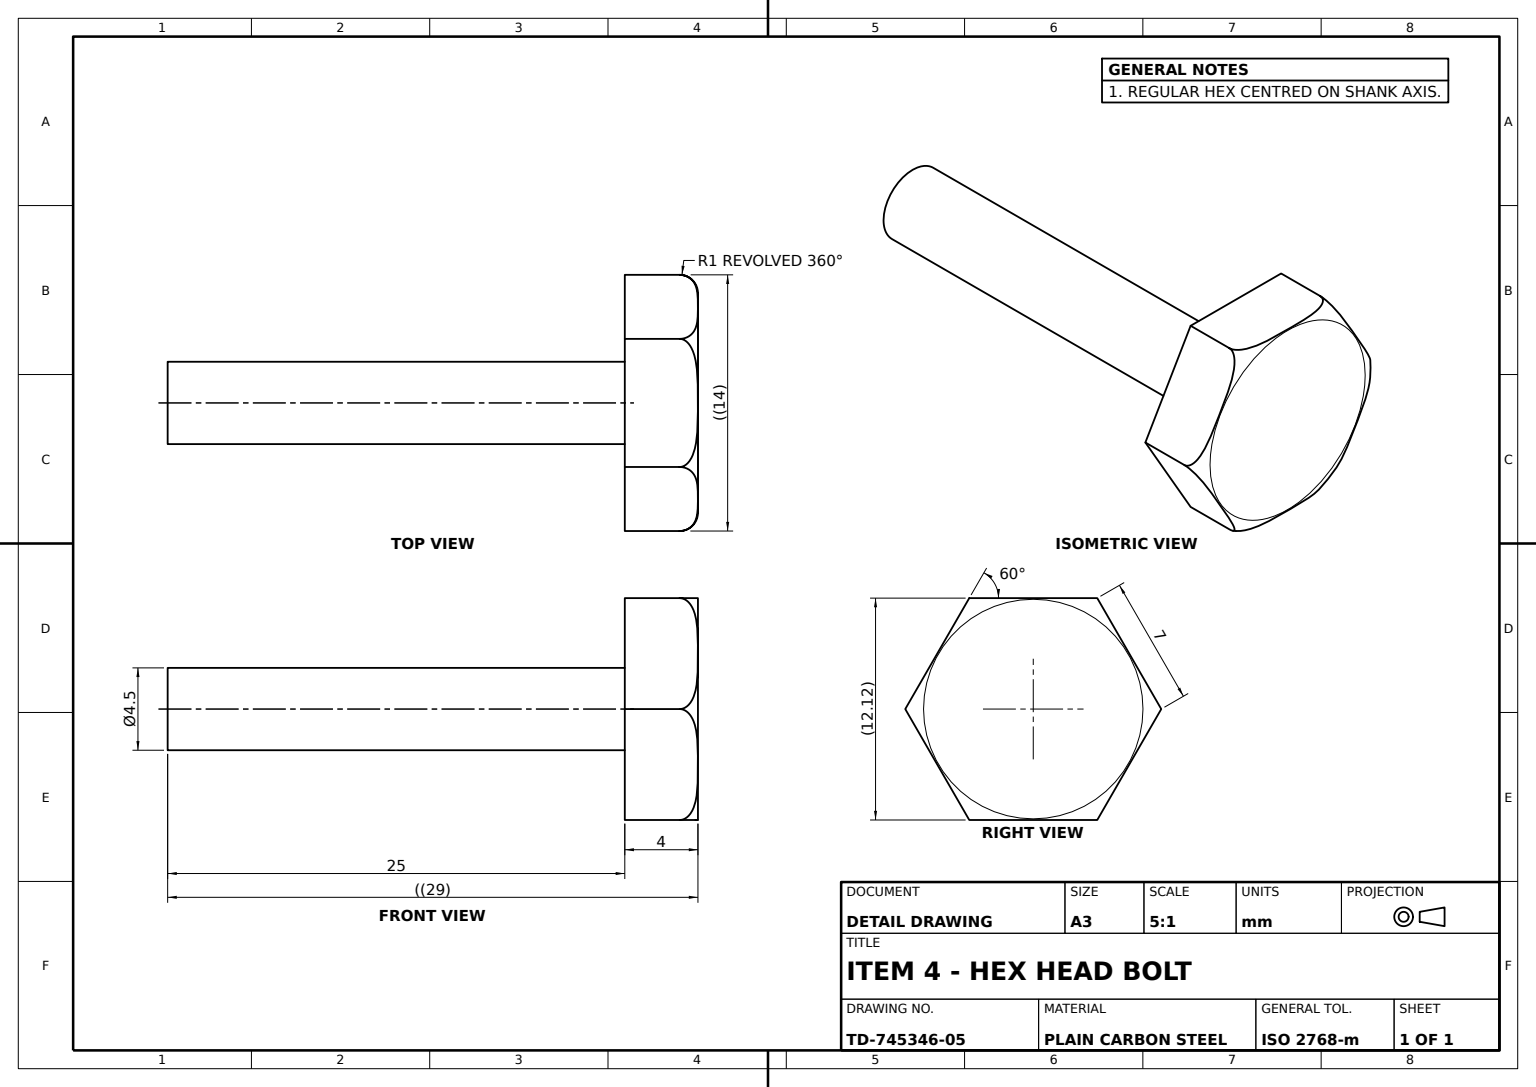
ISO-10303-21;
HEADER;
FILE_DESCRIPTION((''),'2;1');
FILE_NAME('','',(''),(''),'','','');
FILE_SCHEMA(('AUTOMOTIVE_DESIGN'));
ENDSEC;
DATA;
#1=APPLICATION_CONTEXT('');
#2=PRODUCT_CONTEXT('',#1,'mechanical');
#3=PRODUCT('','','',(#2));
#4=PRODUCT_DEFINITION_FORMATION('','',#3);
#5=PRODUCT_DEFINITION_CONTEXT('',#1,'design');
#6=PRODUCT_DEFINITION('','',#4,#5);
#7=PRODUCT_DEFINITION_SHAPE('','',#6);
#8=(LENGTH_UNIT()NAMED_UNIT(*)SI_UNIT(.MILLI.,.METRE.));
#9=(NAMED_UNIT(*)PLANE_ANGLE_UNIT()SI_UNIT($,.RADIAN.));
#10=(NAMED_UNIT(*)SI_UNIT($,.STERADIAN.)SOLID_ANGLE_UNIT());
#11=UNCERTAINTY_MEASURE_WITH_UNIT(LENGTH_MEASURE(1.E-05),#8,'distance_accuracy_value','');
#12=(GEOMETRIC_REPRESENTATION_CONTEXT(3)GLOBAL_UNCERTAINTY_ASSIGNED_CONTEXT((#11))GLOBAL_UNIT_ASSIGNED_CONTEXT((#8,#9,#10))REPRESENTATION_CONTEXT('',''));
#13=CARTESIAN_POINT('',(7.,0.,1.));
#14=VERTEX_POINT('',#13);
#15=CARTESIAN_POINT('',(3.5,-6.062178,1.));
#16=VERTEX_POINT('',#15);
#17=CARTESIAN_POINT('',(7.,0.,0.916819));
#18=CARTESIAN_POINT('',(6.989359,-0.018431,0.835633));
#19=CARTESIAN_POINT('',(6.952796,-0.081759,0.688304));
#20=CARTESIAN_POINT('',(6.92705,-0.126354,0.62203));
#21=CARTESIAN_POINT('',(6.868894,-0.227082,0.507162));
#22=CARTESIAN_POINT('',(6.835753,-0.284484,0.456904));
#23=CARTESIAN_POINT('',(6.766475,-0.404478,0.369773));
#24=CARTESIAN_POINT('',(6.730234,-0.467249,0.332584));
#25=CARTESIAN_POINT('',(6.618164,-0.661359,0.234345));
#26=CARTESIAN_POINT('',(6.539075,-0.798346,0.186761));
#27=CARTESIAN_POINT('',(6.381172,-1.071841,0.114066));
#28=CARTESIAN_POINT('',(6.3014,-1.210012,0.088523));
#29=CARTESIAN_POINT('',(6.060644,-1.627012,0.030791));
#30=CARTESIAN_POINT('',(5.89805,-1.908634,0.017016));
#31=CARTESIAN_POINT('',(5.573222,-2.471253,0.002538));
#32=CARTESIAN_POINT('',(5.41077,-2.752627,0.001924));
#33=CARTESIAN_POINT('',(5.08586,-3.315387,0.001946));
#34=CARTESIAN_POINT('',(4.923388,-3.596798,0.002584));
#35=CARTESIAN_POINT('',(4.598584,-4.159374,0.017273));
#36=CARTESIAN_POINT('',(4.436097,-4.44081,0.031131));
#37=CARTESIAN_POINT('',(4.194192,-4.859802,0.089809));
#38=CARTESIAN_POINT('',(4.113909,-4.998856,0.11589));
#39=CARTESIAN_POINT('',(3.956497,-5.271502,0.189267));
#40=CARTESIAN_POINT('',(3.879027,-5.405684,0.236251));
#41=CARTESIAN_POINT('',(3.729524,-5.66463,0.368438));
#42=CARTESIAN_POINT('',(3.65803,-5.788462,0.453009));
#43=CARTESIAN_POINT('',(3.571901,-5.937642,0.624608));
#44=CARTESIAN_POINT('',(3.546488,-5.981658,0.690617));
#45=CARTESIAN_POINT('',(3.510498,-6.043995,0.836797));
#46=CARTESIAN_POINT('',(3.5,-6.062178,0.917467));
#47=B_SPLINE_CURVE_WITH_KNOTS('',3,(#13,#17,#18,#19,#20,#21,#22,#23,#24,#25,#26,#27,#28,#29,#30,#31,#32,#33,#34,#35,#36,#37,#38,#39,#40,#41,#42,#43,#44,#45,#46,#15),.UNSPECIFIED.,.F.,.F.,(4,2,2,2,2,2,2,2,2,2,2,2,2,2,2,4),(0.000000197,0.000245943,0.000491689,0.000737435,0.000983181,0.001474674,0.001966166,0.00294915,0.003932135,0.004915119,0.005898103,0.006389596,0.006881088,0.00737258,0.007618326,0.007864072),.UNSPECIFIED.);
#48=EDGE_CURVE('',#14,#16,#47,.T.);
#49=ORIENTED_EDGE('',*,*,#48,.F.);
#50=CARTESIAN_POINT('',(7.,0.,4.));
#51=VERTEX_POINT('',#50);
#52=DIRECTION('',(0.,0.,-1.));
#53=VECTOR('',#52,1000.);
#54=LINE('',#50,#53);
#55=EDGE_CURVE('',#51,#14,#54,.T.);
#56=ORIENTED_EDGE('',*,*,#55,.F.);
#57=CARTESIAN_POINT('',(3.5,-6.062178,4.));
#58=VERTEX_POINT('',#57);
#59=DIRECTION('',(0.5,0.866025404,0.));
#60=VECTOR('',#59,1000.);
#61=LINE('',#57,#60);
#62=EDGE_CURVE('',#58,#51,#61,.T.);
#63=ORIENTED_EDGE('',*,*,#62,.F.);
#64=LINE('',#57,#53);
#65=EDGE_CURVE('',#58,#16,#64,.T.);
#66=ORIENTED_EDGE('',*,*,#65,.T.);
#67=EDGE_LOOP('',(#49,#56,#63,#66));
#68=FACE_OUTER_BOUND('',#67,.T.);
#69=DIRECTION('',(-0.866025404,0.5,0.));
#70=DIRECTION('',(-0.5,-0.866025404,0.));
#71=AXIS2_PLACEMENT_3D('',#57,#69,#70);
#72=PLANE('',#71);
#73=ADVANCED_FACE('',(#68),#72,.F.);
#74=CARTESIAN_POINT('',(-6.,0.,0.));
#75=VERTEX_POINT('',#74);
#76=CARTESIAN_POINT('',(6.,0.,0.));
#77=VERTEX_POINT('',#76);
#78=CARTESIAN_POINT('',(0.,0.,0.));
#79=DIRECTION('',(-1.,0.,0.));
#80=AXIS2_PLACEMENT_3D('',#78,#52,#79);
#81=CIRCLE('',#80,6.);
#82=EDGE_CURVE('',#75,#77,#81,.T.);
#83=ORIENTED_EDGE('',*,*,#82,.F.);
#84=CARTESIAN_POINT('',(-7.,0.,1.));
#85=VERTEX_POINT('',#84);
#86=CARTESIAN_POINT('',(-6.,0.,1.));
#87=DIRECTION('',(0.,-1.,0.));
#88=AXIS2_PLACEMENT_3D('',#86,#87,#52);
#89=CIRCLE('',#88,1.);
#90=EDGE_CURVE('',#85,#75,#89,.T.);
#91=ORIENTED_EDGE('',*,*,#90,.F.);
#92=CARTESIAN_POINT('',(-3.5,6.062178,1.));
#93=VERTEX_POINT('',#92);
#94=CARTESIAN_POINT('',(-7.,0.,0.916819));
#95=CARTESIAN_POINT('',(-6.989359,0.018431,0.835633));
#96=CARTESIAN_POINT('',(-6.952796,0.081759,0.688304));
#97=CARTESIAN_POINT('',(-6.92705,0.126354,0.62203));
#98=CARTESIAN_POINT('',(-6.868894,0.227082,0.507162));
#99=CARTESIAN_POINT('',(-6.835753,0.284484,0.456904));
#100=CARTESIAN_POINT('',(-6.766475,0.404478,0.369773));
#101=CARTESIAN_POINT('',(-6.730234,0.467249,0.332584));
#102=CARTESIAN_POINT('',(-6.618164,0.661359,0.234345));
#103=CARTESIAN_POINT('',(-6.539075,0.798346,0.186761));
#104=CARTESIAN_POINT('',(-6.381172,1.071841,0.114066));
#105=CARTESIAN_POINT('',(-6.3014,1.210012,0.088523));
#106=CARTESIAN_POINT('',(-6.060644,1.627012,0.030791));
#107=CARTESIAN_POINT('',(-5.89805,1.908634,0.017016));
#108=CARTESIAN_POINT('',(-5.573222,2.471253,0.002538));
#109=CARTESIAN_POINT('',(-5.41077,2.752627,0.001924));
#110=CARTESIAN_POINT('',(-5.08586,3.315387,0.001946));
#111=CARTESIAN_POINT('',(-4.923388,3.596798,0.002584));
#112=CARTESIAN_POINT('',(-4.598584,4.159374,0.017273));
#113=CARTESIAN_POINT('',(-4.436097,4.44081,0.031131));
#114=CARTESIAN_POINT('',(-4.194192,4.859802,0.089809));
#115=CARTESIAN_POINT('',(-4.113909,4.998856,0.11589));
#116=CARTESIAN_POINT('',(-3.956497,5.271502,0.189267));
#117=CARTESIAN_POINT('',(-3.879027,5.405684,0.236251));
#118=CARTESIAN_POINT('',(-3.729524,5.66463,0.368438));
#119=CARTESIAN_POINT('',(-3.65803,5.788462,0.453009));
#120=CARTESIAN_POINT('',(-3.571901,5.937642,0.624608));
#121=CARTESIAN_POINT('',(-3.546488,5.981658,0.690617));
#122=CARTESIAN_POINT('',(-3.510498,6.043995,0.836797));
#123=CARTESIAN_POINT('',(-3.5,6.062178,0.917467));
#124=B_SPLINE_CURVE_WITH_KNOTS('',3,(#84,#94,#95,#96,#97,#98,#99,#100,#101,#102,#103,#104,#105,#106,#107,#108,#109,#110,#111,#112,#113,#114,#115,#116,#117,#118,#119,#120,#121,#122,#123,#92),.UNSPECIFIED.,.F.,.F.,(4,2,2,2,2,2,2,2,2,2,2,2,2,2,2,4),(0.000000197,0.000245943,0.000491689,0.000737435,0.000983181,0.001474674,0.001966166,0.00294915,0.003932135,0.004915119,0.005898103,0.006389596,0.006881088,0.00737258,0.007618326,0.007864072),.UNSPECIFIED.);
#125=EDGE_CURVE('',#85,#93,#124,.T.);
#126=ORIENTED_EDGE('',*,*,#125,.T.);
#127=CARTESIAN_POINT('',(3.5,6.062178,1.));
#128=VERTEX_POINT('',#127);
#129=CARTESIAN_POINT('',(-3.5,6.062178,0.918745));
#130=CARTESIAN_POINT('',(-3.479253,6.062178,0.837184));
#131=CARTESIAN_POINT('',(-3.406434,6.062178,0.689536));
#132=CARTESIAN_POINT('',(-3.356443,6.062178,0.624754));
#133=CARTESIAN_POINT('',(-3.181801,6.062178,0.451074));
#134=CARTESIAN_POINT('',(-3.039481,6.062178,0.367715));
#135=CARTESIAN_POINT('',(-2.741948,6.062178,0.236325));
#136=CARTESIAN_POINT('',(-2.587351,6.062178,0.189346));
#137=CARTESIAN_POINT('',(-2.271801,6.062178,0.115802));
#138=CARTESIAN_POINT('',(-2.110688,6.062178,0.08969));
#139=CARTESIAN_POINT('',(-1.628975,6.062178,0.031285));
#140=CARTESIAN_POINT('',(-1.306565,6.062178,0.01745));
#141=CARTESIAN_POINT('',(-0.661096,6.062178,0.002671));
#142=CARTESIAN_POINT('',(-0.338023,6.062178,0.001986));
#143=CARTESIAN_POINT('',(0.146635,6.062178,0.001911));
#144=CARTESIAN_POINT('',(0.310793,6.062178,0.002231));
#145=CARTESIAN_POINT('',(0.636565,6.062178,0.004285));
#146=CARTESIAN_POINT('',(0.799424,6.062178,0.00602));
#147=CARTESIAN_POINT('',(1.287798,6.062178,0.016692));
#148=CARTESIAN_POINT('',(1.613148,6.062178,0.03008));
#149=CARTESIAN_POINT('',(2.09976,6.062178,0.088029));
#150=CARTESIAN_POINT('',(2.260961,6.062178,0.11381));
#151=CARTESIAN_POINT('',(2.576967,6.062178,0.186427));
#152=CARTESIAN_POINT('',(2.73221,6.062178,0.232886));
#153=CARTESIAN_POINT('',(3.032378,6.062178,0.363764));
#154=CARTESIAN_POINT('',(3.176959,6.062178,0.447407));
#155=CARTESIAN_POINT('',(3.354082,6.062178,0.621855));
#156=CARTESIAN_POINT('',(3.405203,6.062178,0.68762));
#157=CARTESIAN_POINT('',(3.478814,6.062178,0.835728));
#158=CARTESIAN_POINT('',(3.5,6.062178,0.918017));
#159=B_SPLINE_CURVE_WITH_KNOTS('',3,(#92,#129,#130,#131,#132,#133,#134,#135,#136,#137,#138,#139,#140,#141,#142,#143,#144,#145,#146,#147,#148,#149,#150,#151,#152,#153,#154,#155,#156,#157,#158,#127),.UNSPECIFIED.,.F.,.F.,(4,2,2,2,2,2,2,2,2,2,2,2,2,2,2,4),(0.011690306,0.011934522,0.012178739,0.012667172,0.013155605,0.013644038,0.014620904,0.01559777,0.016086203,0.016574636,0.017551502,0.018039935,0.018528368,0.019016801,0.019261017,0.019505234),.UNSPECIFIED.);
#160=EDGE_CURVE('',#93,#128,#159,.T.);
#161=ORIENTED_EDGE('',*,*,#160,.T.);
#162=CARTESIAN_POINT('',(3.5,6.062178,0.916819));
#163=CARTESIAN_POINT('',(3.510641,6.043747,0.835633));
#164=CARTESIAN_POINT('',(3.547204,5.980418,0.688304));
#165=CARTESIAN_POINT('',(3.57295,5.935824,0.62203));
#166=CARTESIAN_POINT('',(3.631106,5.835096,0.507162));
#167=CARTESIAN_POINT('',(3.664247,5.777694,0.456904));
#168=CARTESIAN_POINT('',(3.733525,5.6577,0.369773));
#169=CARTESIAN_POINT('',(3.769766,5.594929,0.332584));
#170=CARTESIAN_POINT('',(3.881836,5.400819,0.234345));
#171=CARTESIAN_POINT('',(3.960925,5.263832,0.186761));
#172=CARTESIAN_POINT('',(4.118828,4.990337,0.114066));
#173=CARTESIAN_POINT('',(4.1986,4.852166,0.088523));
#174=CARTESIAN_POINT('',(4.439356,4.435166,0.030791));
#175=CARTESIAN_POINT('',(4.60195,4.153544,0.017016));
#176=CARTESIAN_POINT('',(4.926778,3.590925,0.002538));
#177=CARTESIAN_POINT('',(5.08923,3.309551,0.001924));
#178=CARTESIAN_POINT('',(5.41414,2.746791,0.001946));
#179=CARTESIAN_POINT('',(5.576612,2.46538,0.002584));
#180=CARTESIAN_POINT('',(5.901416,1.902804,0.017273));
#181=CARTESIAN_POINT('',(6.063903,1.621368,0.031131));
#182=CARTESIAN_POINT('',(6.305808,1.202376,0.089809));
#183=CARTESIAN_POINT('',(6.386091,1.063322,0.11589));
#184=CARTESIAN_POINT('',(6.543503,0.790676,0.189267));
#185=CARTESIAN_POINT('',(6.620973,0.656494,0.236251));
#186=CARTESIAN_POINT('',(6.770476,0.397548,0.368438));
#187=CARTESIAN_POINT('',(6.84197,0.273716,0.453009));
#188=CARTESIAN_POINT('',(6.928099,0.124536,0.624608));
#189=CARTESIAN_POINT('',(6.953512,0.080519,0.690617));
#190=CARTESIAN_POINT('',(6.989502,0.018183,0.836797));
#191=CARTESIAN_POINT('',(7.,0.,0.917467));
#192=B_SPLINE_CURVE_WITH_KNOTS('',3,(#127,#162,#163,#164,#165,#166,#167,#168,#169,#170,#171,#172,#173,#174,#175,#176,#177,#178,#179,#180,#181,#182,#183,#184,#185,#186,#187,#188,#189,#190,#191,#13),.UNSPECIFIED.,.F.,.F.,(4,2,2,2,2,2,2,2,2,2,2,2,2,2,2,4),(0.000000197,0.000245943,0.000491689,0.000737435,0.000983181,0.001474674,0.001966166,0.00294915,0.003932135,0.004915119,0.005898103,0.006389596,0.006881088,0.00737258,0.007618326,0.007864072),.UNSPECIFIED.);
#193=EDGE_CURVE('',#128,#14,#192,.T.);
#194=ORIENTED_EDGE('',*,*,#193,.T.);
#195=CARTESIAN_POINT('',(6.,0.,1.));
#196=DIRECTION('',(0.,1.,0.));
#197=AXIS2_PLACEMENT_3D('',#195,#196,#79);
#198=CIRCLE('',#197,1.);
#199=EDGE_CURVE('',#14,#77,#198,.T.);
#200=ORIENTED_EDGE('',*,*,#199,.T.);
#201=EDGE_LOOP('',(#83,#91,#126,#161,#194,#200));
#202=FACE_OUTER_BOUND('',#201,.T.);
#203=CARTESIAN_POINT('',(0.,0.,1.));
#204=AXIS2_PLACEMENT_3D('',#203,#52,#79);
#205=TOROIDAL_SURFACE('',#204,6.,1.);
#206=ADVANCED_FACE('',(#202),#205,.T.);
#207=CARTESIAN_POINT('',(3.5,6.062178,4.));
#208=VERTEX_POINT('',#207);
#209=LINE('',#207,#53);
#210=EDGE_CURVE('',#208,#128,#209,.T.);
#211=ORIENTED_EDGE('',*,*,#210,.T.);
#212=ORIENTED_EDGE('',*,*,#160,.F.);
#213=CARTESIAN_POINT('',(-3.5,6.062178,4.));
#214=VERTEX_POINT('',#213);
#215=LINE('',#213,#53);
#216=EDGE_CURVE('',#214,#93,#215,.T.);
#217=ORIENTED_EDGE('',*,*,#216,.F.);
#218=VECTOR('',#79,1000.);
#219=LINE('',#207,#218);
#220=EDGE_CURVE('',#208,#214,#219,.T.);
#221=ORIENTED_EDGE('',*,*,#220,.F.);
#222=EDGE_LOOP('',(#211,#212,#217,#221));
#223=FACE_OUTER_BOUND('',#222,.T.);
#224=AXIS2_PLACEMENT_3D('',#207,#87,#52);
#225=PLANE('',#224);
#226=ADVANCED_FACE('',(#223),#225,.F.);
#227=ORIENTED_EDGE('',*,*,#193,.F.);
#228=ORIENTED_EDGE('',*,*,#210,.F.);
#229=DIRECTION('',(-0.5,0.866025404,0.));
#230=VECTOR('',#229,1000.);
#231=LINE('',#50,#230);
#232=EDGE_CURVE('',#51,#208,#231,.T.);
#233=ORIENTED_EDGE('',*,*,#232,.F.);
#234=ORIENTED_EDGE('',*,*,#55,.T.);
#235=EDGE_LOOP('',(#227,#228,#233,#234));
#236=FACE_OUTER_BOUND('',#235,.T.);
#237=DIRECTION('',(-0.866025404,-0.5,0.));
#238=DIRECTION('',(0.5,-0.866025404,0.));
#239=AXIS2_PLACEMENT_3D('',#50,#237,#238);
#240=PLANE('',#239);
#241=ADVANCED_FACE('',(#236),#240,.F.);
#242=CARTESIAN_POINT('',(-2.25,0.,29.));
#243=VERTEX_POINT('',#242);
#244=CARTESIAN_POINT('',(2.25,0.,29.));
#245=VERTEX_POINT('',#244);
#246=CARTESIAN_POINT('',(0.,0.,29.));
#247=DIRECTION('',(0.,0.,1.));
#248=DIRECTION('',(1.,0.,0.));
#249=AXIS2_PLACEMENT_3D('',#246,#247,#248);
#250=CIRCLE('',#249,2.25);
#251=EDGE_CURVE('',#243,#245,#250,.T.);
#252=ORIENTED_EDGE('',*,*,#251,.T.);
#253=EDGE_CURVE('',#245,#243,#250,.T.);
#254=ORIENTED_EDGE('',*,*,#253,.T.);
#255=EDGE_LOOP('',(#252,#254));
#256=FACE_OUTER_BOUND('',#255,.T.);
#257=PLANE('',#249);
#258=ADVANCED_FACE('',(#256),#257,.T.);
#259=ORIENTED_EDGE('',*,*,#65,.F.);
#260=CARTESIAN_POINT('',(-3.5,-6.062178,4.));
#261=VERTEX_POINT('',#260);
#262=VECTOR('',#248,1000.);
#263=LINE('',#260,#262);
#264=EDGE_CURVE('',#261,#58,#263,.T.);
#265=ORIENTED_EDGE('',*,*,#264,.F.);
#266=CARTESIAN_POINT('',(-3.5,-6.062178,1.));
#267=VERTEX_POINT('',#266);
#268=LINE('',#260,#53);
#269=EDGE_CURVE('',#261,#267,#268,.T.);
#270=ORIENTED_EDGE('',*,*,#269,.T.);
#271=CARTESIAN_POINT('',(3.5,-6.062178,0.918745));
#272=CARTESIAN_POINT('',(3.479253,-6.062178,0.837184));
#273=CARTESIAN_POINT('',(3.406434,-6.062178,0.689536));
#274=CARTESIAN_POINT('',(3.356443,-6.062178,0.624754));
#275=CARTESIAN_POINT('',(3.181801,-6.062178,0.451074));
#276=CARTESIAN_POINT('',(3.039481,-6.062178,0.367715));
#277=CARTESIAN_POINT('',(2.741948,-6.062178,0.236325));
#278=CARTESIAN_POINT('',(2.587351,-6.062178,0.189346));
#279=CARTESIAN_POINT('',(2.271801,-6.062178,0.115802));
#280=CARTESIAN_POINT('',(2.110688,-6.062178,0.08969));
#281=CARTESIAN_POINT('',(1.628975,-6.062178,0.031285));
#282=CARTESIAN_POINT('',(1.306565,-6.062178,0.01745));
#283=CARTESIAN_POINT('',(0.661096,-6.062178,0.002671));
#284=CARTESIAN_POINT('',(0.338023,-6.062178,0.001986));
#285=CARTESIAN_POINT('',(-0.146635,-6.062178,0.001911));
#286=CARTESIAN_POINT('',(-0.310793,-6.062178,0.002231));
#287=CARTESIAN_POINT('',(-0.636565,-6.062178,0.004285));
#288=CARTESIAN_POINT('',(-0.799424,-6.062178,0.00602));
#289=CARTESIAN_POINT('',(-1.287798,-6.062178,0.016692));
#290=CARTESIAN_POINT('',(-1.613148,-6.062178,0.03008));
#291=CARTESIAN_POINT('',(-2.09976,-6.062178,0.088029));
#292=CARTESIAN_POINT('',(-2.260961,-6.062178,0.11381));
#293=CARTESIAN_POINT('',(-2.576967,-6.062178,0.186427));
#294=CARTESIAN_POINT('',(-2.73221,-6.062178,0.232886));
#295=CARTESIAN_POINT('',(-3.032378,-6.062178,0.363764));
#296=CARTESIAN_POINT('',(-3.176959,-6.062178,0.447407));
#297=CARTESIAN_POINT('',(-3.354082,-6.062178,0.621855));
#298=CARTESIAN_POINT('',(-3.405203,-6.062178,0.68762));
#299=CARTESIAN_POINT('',(-3.478814,-6.062178,0.835728));
#300=CARTESIAN_POINT('',(-3.5,-6.062178,0.918017));
#301=B_SPLINE_CURVE_WITH_KNOTS('',3,(#15,#271,#272,#273,#274,#275,#276,#277,#278,#279,#280,#281,#282,#283,#284,#285,#286,#287,#288,#289,#290,#291,#292,#293,#294,#295,#296,#297,#298,#299,#300,#266),.UNSPECIFIED.,.F.,.F.,(4,2,2,2,2,2,2,2,2,2,2,2,2,2,2,4),(0.011690306,0.011934522,0.012178739,0.012667172,0.013155605,0.013644038,0.014620904,0.01559777,0.016086203,0.016574636,0.017551502,0.018039935,0.018528368,0.019016801,0.019261017,0.019505234),.UNSPECIFIED.);
#302=EDGE_CURVE('',#16,#267,#301,.T.);
#303=ORIENTED_EDGE('',*,*,#302,.F.);
#304=EDGE_LOOP('',(#259,#265,#270,#303));
#305=FACE_OUTER_BOUND('',#304,.T.);
#306=AXIS2_PLACEMENT_3D('',#260,#196,#79);
#307=PLANE('',#306);
#308=ADVANCED_FACE('',(#305),#307,.F.);
#309=CARTESIAN_POINT('',(-2.25,0.,4.));
#310=VERTEX_POINT('',#309);
#311=CARTESIAN_POINT('',(2.25,0.,4.));
#312=VERTEX_POINT('',#311);
#313=CARTESIAN_POINT('',(0.,0.,4.));
#314=AXIS2_PLACEMENT_3D('',#313,#247,#248);
#315=CIRCLE('',#314,2.25);
#316=EDGE_CURVE('',#310,#312,#315,.T.);
#317=ORIENTED_EDGE('',*,*,#316,.F.);
#318=EDGE_CURVE('',#312,#310,#315,.T.);
#319=ORIENTED_EDGE('',*,*,#318,.F.);
#320=EDGE_LOOP('',(#317,#319));
#321=FACE_BOUND('',#320,.T.);
#322=CARTESIAN_POINT('',(-7.,0.,4.));
#323=VERTEX_POINT('',#322);
#324=VECTOR('',#70,1000.);
#325=LINE('',#213,#324);
#326=EDGE_CURVE('',#214,#323,#325,.T.);
#327=ORIENTED_EDGE('',*,*,#326,.T.);
#328=VECTOR('',#238,1000.);
#329=LINE('',#322,#328);
#330=EDGE_CURVE('',#323,#261,#329,.T.);
#331=ORIENTED_EDGE('',*,*,#330,.T.);
#332=ORIENTED_EDGE('',*,*,#264,.T.);
#333=ORIENTED_EDGE('',*,*,#62,.T.);
#334=ORIENTED_EDGE('',*,*,#232,.T.);
#335=ORIENTED_EDGE('',*,*,#220,.T.);
#336=EDGE_LOOP('',(#327,#331,#332,#333,#334,#335));
#337=FACE_OUTER_BOUND('',#336,.T.);
#338=PLANE('',#314);
#339=ADVANCED_FACE('',(#321,#337),#338,.T.);
#340=ORIENTED_EDGE('',*,*,#302,.T.);
#341=CARTESIAN_POINT('',(-3.5,-6.062178,0.916819));
#342=CARTESIAN_POINT('',(-3.510641,-6.043747,0.835633));
#343=CARTESIAN_POINT('',(-3.547204,-5.980418,0.688304));
#344=CARTESIAN_POINT('',(-3.57295,-5.935824,0.62203));
#345=CARTESIAN_POINT('',(-3.631106,-5.835096,0.507162));
#346=CARTESIAN_POINT('',(-3.664247,-5.777694,0.456904));
#347=CARTESIAN_POINT('',(-3.733525,-5.6577,0.369773));
#348=CARTESIAN_POINT('',(-3.769766,-5.594929,0.332584));
#349=CARTESIAN_POINT('',(-3.881836,-5.400819,0.234345));
#350=CARTESIAN_POINT('',(-3.960925,-5.263832,0.186761));
#351=CARTESIAN_POINT('',(-4.118828,-4.990337,0.114066));
#352=CARTESIAN_POINT('',(-4.1986,-4.852166,0.088523));
#353=CARTESIAN_POINT('',(-4.439356,-4.435166,0.030791));
#354=CARTESIAN_POINT('',(-4.60195,-4.153544,0.017016));
#355=CARTESIAN_POINT('',(-4.926778,-3.590925,0.002538));
#356=CARTESIAN_POINT('',(-5.08923,-3.309551,0.001924));
#357=CARTESIAN_POINT('',(-5.41414,-2.746791,0.001946));
#358=CARTESIAN_POINT('',(-5.576612,-2.46538,0.002584));
#359=CARTESIAN_POINT('',(-5.901416,-1.902804,0.017273));
#360=CARTESIAN_POINT('',(-6.063903,-1.621368,0.031131));
#361=CARTESIAN_POINT('',(-6.305808,-1.202376,0.089809));
#362=CARTESIAN_POINT('',(-6.386091,-1.063322,0.11589));
#363=CARTESIAN_POINT('',(-6.543503,-0.790676,0.189267));
#364=CARTESIAN_POINT('',(-6.620973,-0.656494,0.236251));
#365=CARTESIAN_POINT('',(-6.770476,-0.397548,0.368438));
#366=CARTESIAN_POINT('',(-6.84197,-0.273716,0.453009));
#367=CARTESIAN_POINT('',(-6.928099,-0.124536,0.624608));
#368=CARTESIAN_POINT('',(-6.953512,-0.080519,0.690617));
#369=CARTESIAN_POINT('',(-6.989502,-0.018183,0.836797));
#370=CARTESIAN_POINT('',(-7.,0.,0.917467));
#371=B_SPLINE_CURVE_WITH_KNOTS('',3,(#266,#341,#342,#343,#344,#345,#346,#347,#348,#349,#350,#351,#352,#353,#354,#355,#356,#357,#358,#359,#360,#361,#362,#363,#364,#365,#366,#367,#368,#369,#370,#84),.UNSPECIFIED.,.F.,.F.,(4,2,2,2,2,2,2,2,2,2,2,2,2,2,2,4),(0.000000197,0.000245943,0.000491689,0.000737435,0.000983181,0.001474674,0.001966166,0.00294915,0.003932135,0.004915119,0.005898103,0.006389596,0.006881088,0.00737258,0.007618326,0.007864072),.UNSPECIFIED.);
#372=EDGE_CURVE('',#267,#85,#371,.T.);
#373=ORIENTED_EDGE('',*,*,#372,.T.);
#374=ORIENTED_EDGE('',*,*,#90,.T.);
#375=EDGE_CURVE('',#77,#75,#81,.T.);
#376=ORIENTED_EDGE('',*,*,#375,.F.);
#377=ORIENTED_EDGE('',*,*,#199,.F.);
#378=ORIENTED_EDGE('',*,*,#48,.T.);
#379=EDGE_LOOP('',(#340,#373,#374,#376,#377,#378));
#380=FACE_OUTER_BOUND('',#379,.T.);
#381=ADVANCED_FACE('',(#380),#205,.T.);
#382=LINE('',#244,#53);
#383=EDGE_CURVE('',#245,#312,#382,.T.);
#384=ORIENTED_EDGE('',*,*,#383,.F.);
#385=ORIENTED_EDGE('',*,*,#251,.F.);
#386=LINE('',#242,#53);
#387=EDGE_CURVE('',#243,#310,#386,.T.);
#388=ORIENTED_EDGE('',*,*,#387,.T.);
#389=ORIENTED_EDGE('',*,*,#316,.T.);
#390=EDGE_LOOP('',(#384,#385,#388,#389));
#391=FACE_OUTER_BOUND('',#390,.T.);
#392=AXIS2_PLACEMENT_3D('',#246,#52,#79);
#393=CYLINDRICAL_SURFACE('',#392,2.25);
#394=ADVANCED_FACE('',(#391),#393,.T.);
#395=ORIENTED_EDGE('',*,*,#387,.F.);
#396=ORIENTED_EDGE('',*,*,#253,.F.);
#397=ORIENTED_EDGE('',*,*,#383,.T.);
#398=ORIENTED_EDGE('',*,*,#318,.T.);
#399=EDGE_LOOP('',(#395,#396,#397,#398));
#400=FACE_OUTER_BOUND('',#399,.T.);
#401=ADVANCED_FACE('',(#400),#393,.T.);
#402=ORIENTED_EDGE('',*,*,#125,.F.);
#403=LINE('',#322,#53);
#404=EDGE_CURVE('',#323,#85,#403,.T.);
#405=ORIENTED_EDGE('',*,*,#404,.F.);
#406=ORIENTED_EDGE('',*,*,#326,.F.);
#407=ORIENTED_EDGE('',*,*,#216,.T.);
#408=EDGE_LOOP('',(#402,#405,#406,#407));
#409=FACE_OUTER_BOUND('',#408,.T.);
#410=DIRECTION('',(0.866025404,-0.5,0.));
#411=AXIS2_PLACEMENT_3D('',#213,#410,#59);
#412=PLANE('',#411);
#413=ADVANCED_FACE('',(#409),#412,.F.);
#414=ORIENTED_EDGE('',*,*,#330,.F.);
#415=ORIENTED_EDGE('',*,*,#404,.T.);
#416=ORIENTED_EDGE('',*,*,#372,.F.);
#417=ORIENTED_EDGE('',*,*,#269,.F.);
#418=EDGE_LOOP('',(#414,#415,#416,#417));
#419=FACE_OUTER_BOUND('',#418,.T.);
#420=DIRECTION('',(0.866025404,0.5,0.));
#421=AXIS2_PLACEMENT_3D('',#322,#420,#229);
#422=PLANE('',#421);
#423=ADVANCED_FACE('',(#419),#422,.F.);
#424=ORIENTED_EDGE('',*,*,#82,.T.);
#425=ORIENTED_EDGE('',*,*,#375,.T.);
#426=EDGE_LOOP('',(#424,#425));
#427=FACE_OUTER_BOUND('',#426,.T.);
#428=AXIS2_PLACEMENT_3D('',#78,#247,#248);
#429=PLANE('',#428);
#430=ADVANCED_FACE('',(#427),#429,.F.);
#431=CLOSED_SHELL('',(#73,#206,#226,#241,#258,#308,#339,#381,#394,#401,#413,#423,#430));
#432=MANIFOLD_SOLID_BREP('',#431);
#433=ADVANCED_BREP_SHAPE_REPRESENTATION('',(#432),#12);
#434=SHAPE_DEFINITION_REPRESENTATION(#7,#433);
ENDSEC;
END-ISO-10303-21;
